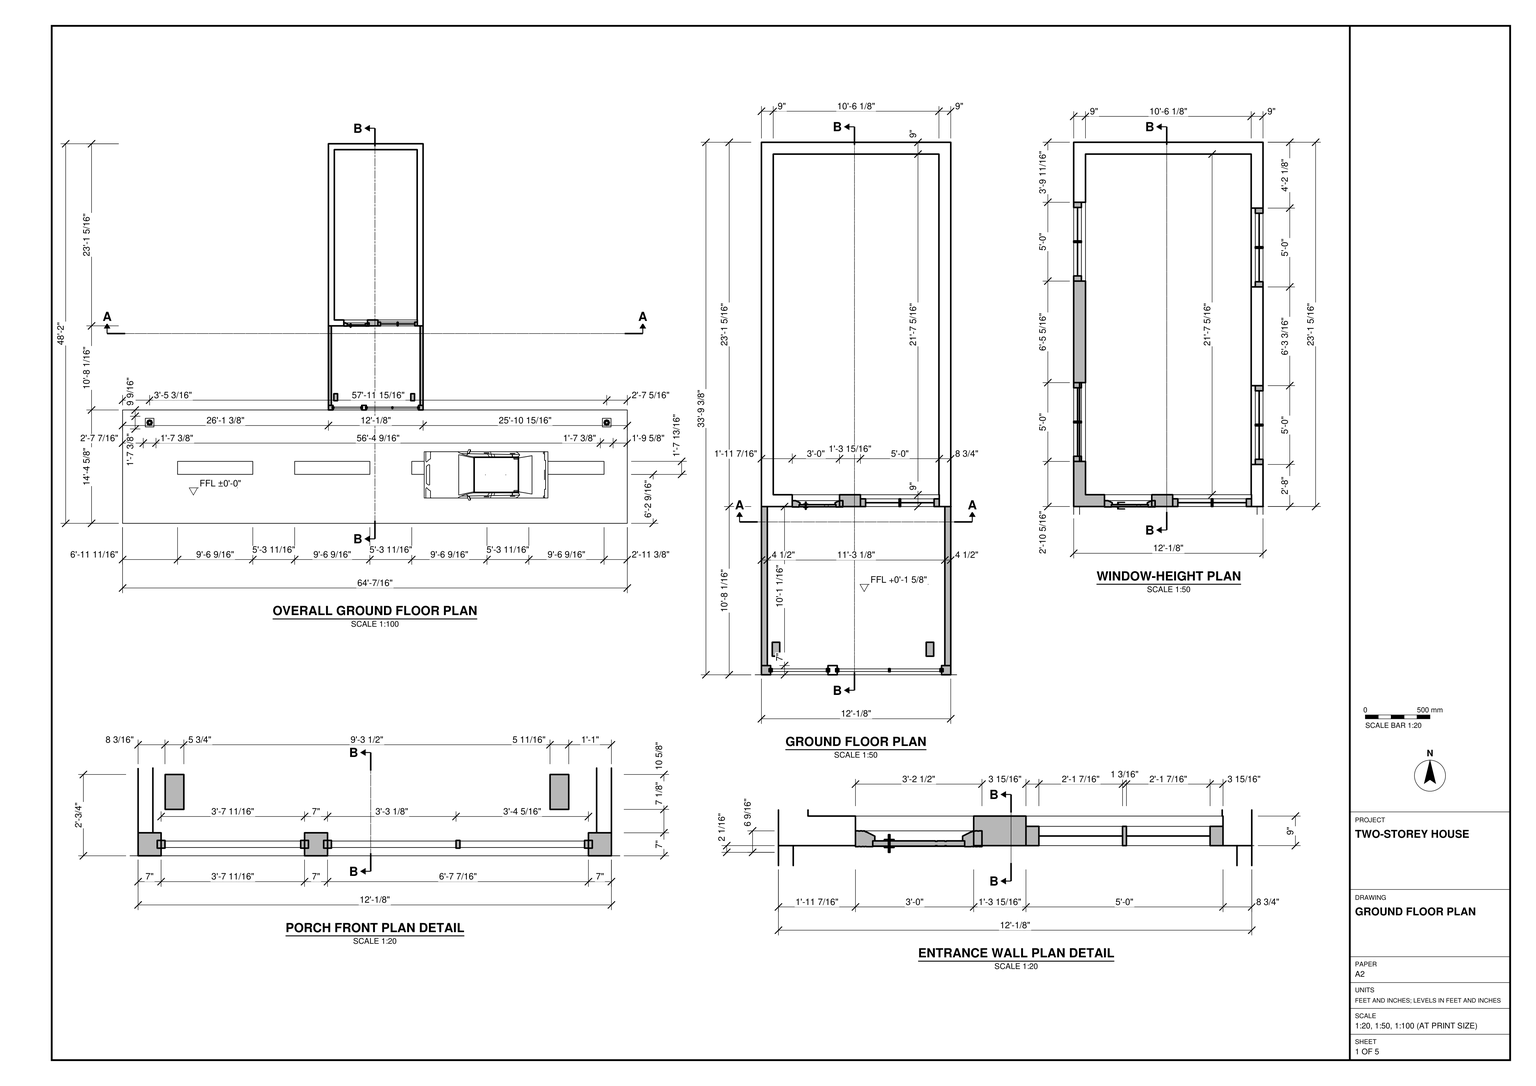
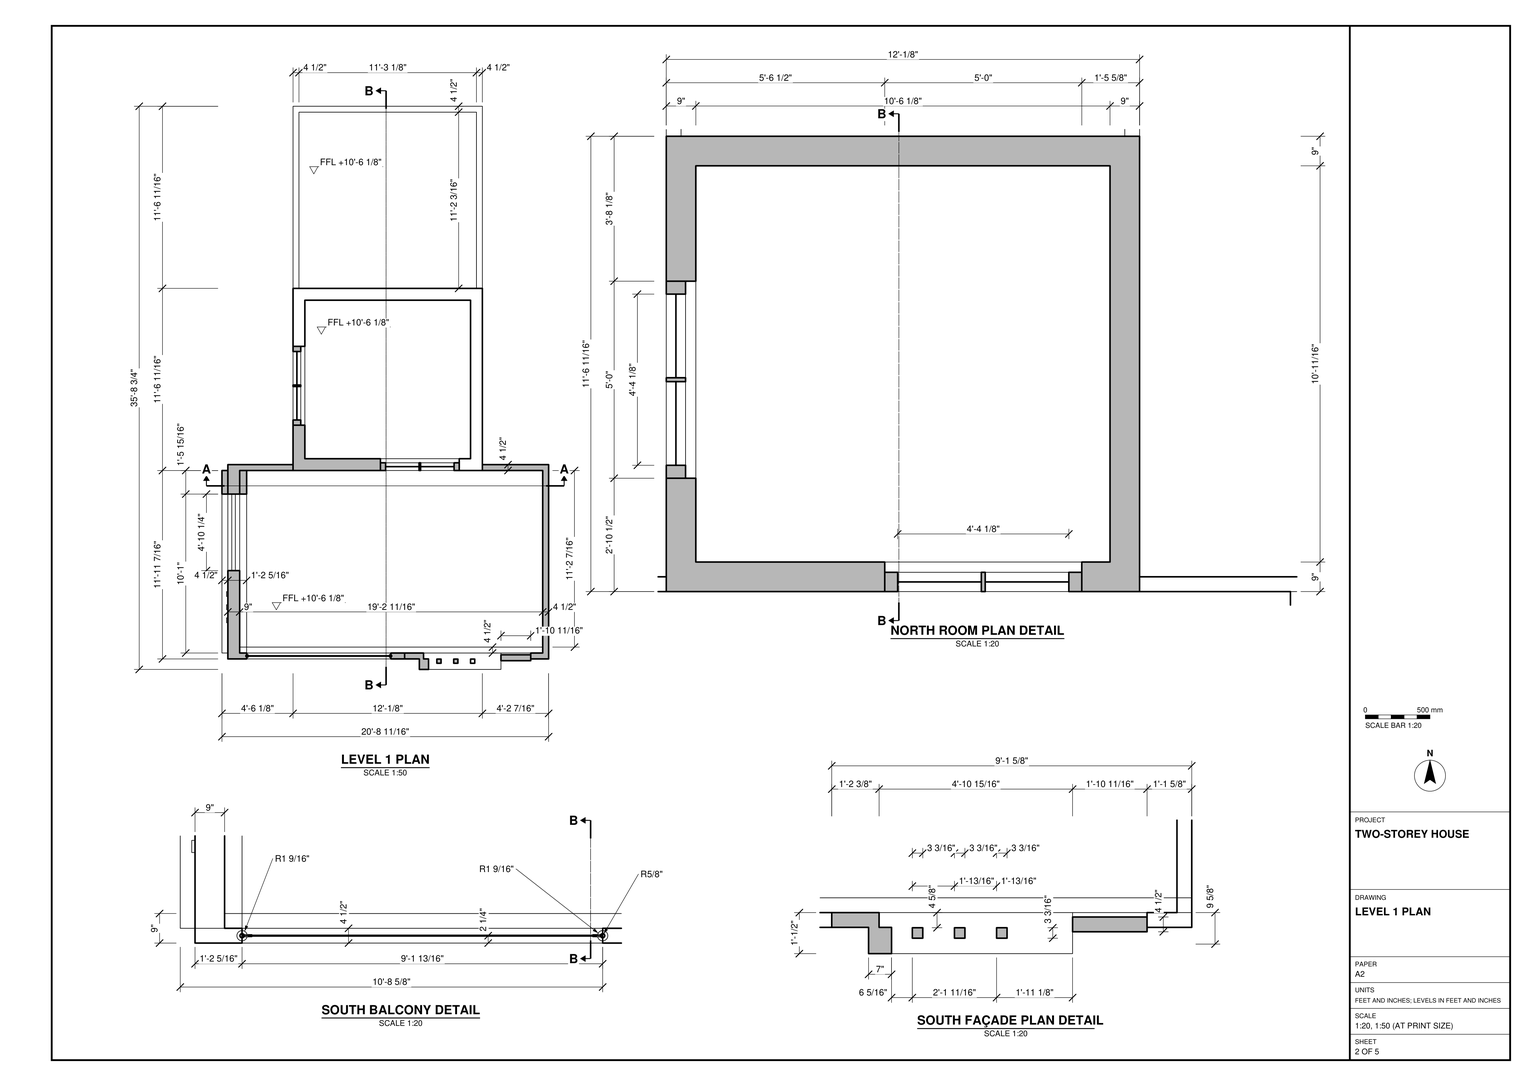
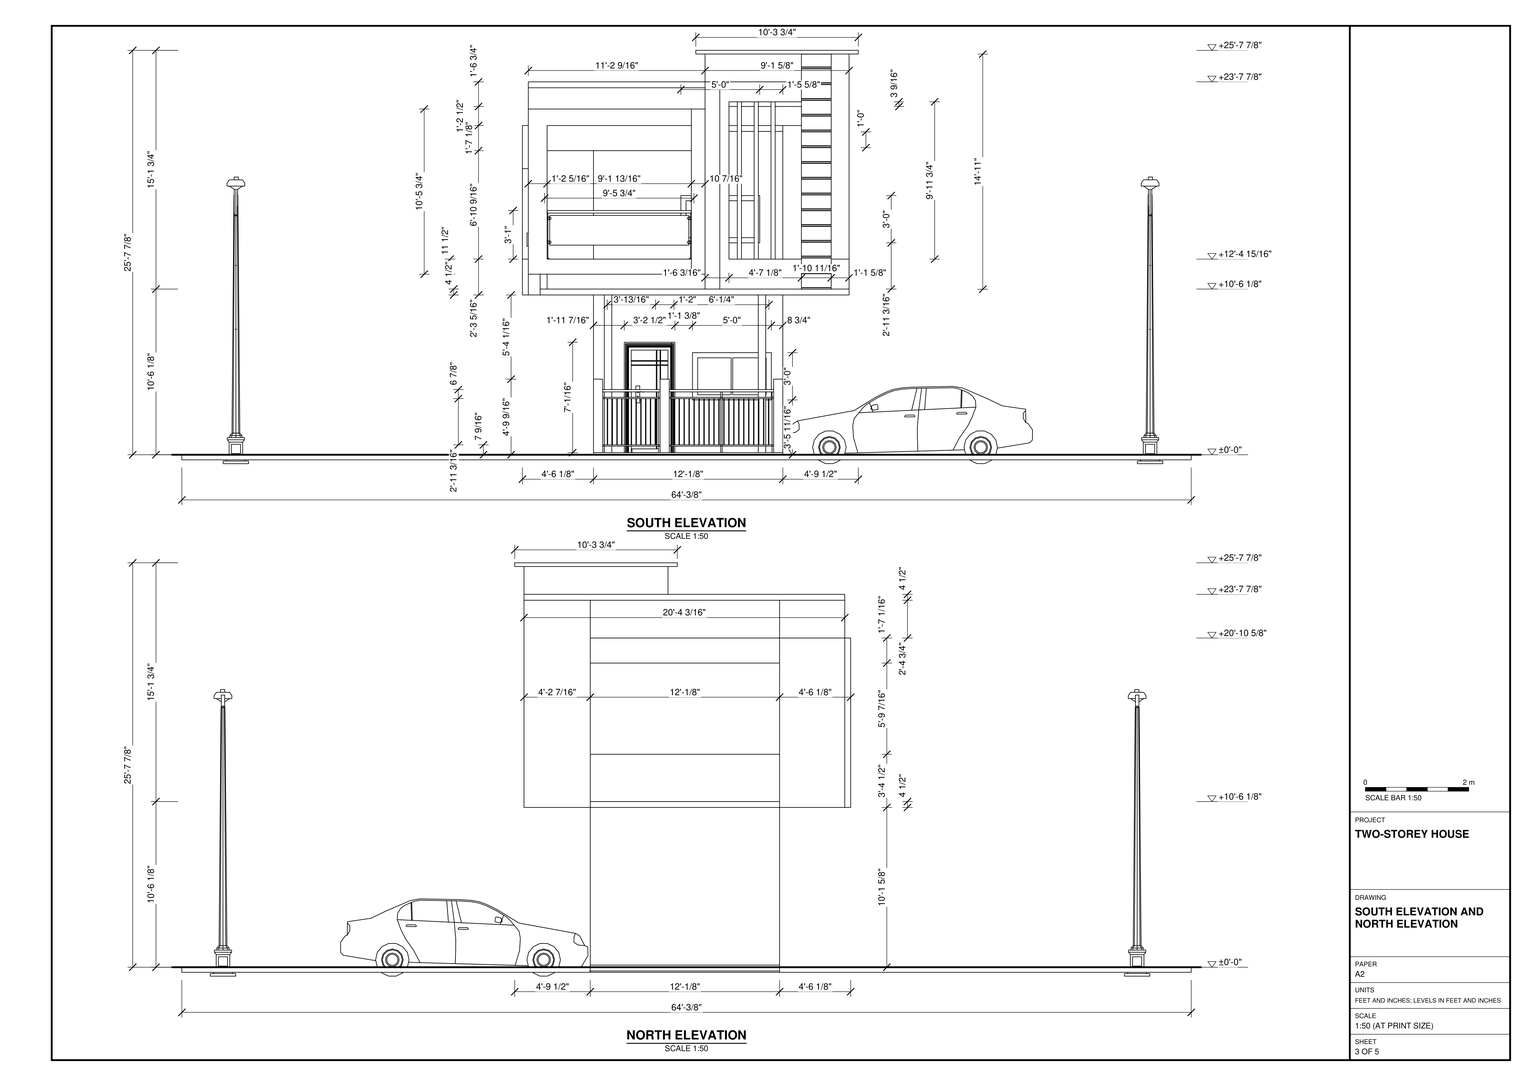
Build the house and its street frontage in SketchUp from task_files/diagram_01.pdf. Work in feet and inches. The complete model, including the street, shall measure 64'-7/16" along X, 48'-2" along Y and 26'-2 11/16" along Z. Use ±0'-0" as the ground-floor datum and +10'-6 1/8" as the upper-floor level.

Set the narrow ground-floor room perpendicular to the street, with the covered porch between the entrance wall and the road. Model the slabs, the 9" room walls, the framed door and windows, and the porch posts and railing. Use the window-height plan to locate the openings along both sides. On the upper floor, extend the wider south portion beyond both sides of the porch and retain the narrower room and terrace to the north. Follow the plan details for wall and parapet thicknesses. Reproduce the recessed south balcony, its guard, the adjacent vertical façade members and horizontal bands, and the stepped flat roofline.

Include the road markings, the car and the street lamps in the positions shown. Decor and loose items may be any suitable library components. Keep shell elements such as walls, slabs and roofs, and each furniture or joinery piece shown, in separate groups or components; use components for repeated parts. Save one SketchUp model as output_files/two_storey_house_with_a_balcony_and_street_frontage.skp.

# SketchUp Ruby script. Lengths in inches.
U = 1.inch
M = Sketchup.active_model
def pt(a) = Geom::Point3d.new(a.map { |v| v * U })
def face(e, loops, mat)
  f = e.add_face(loops[0].map { |a| pt(a) })
  loops[1..].each { |l| e.add_face(l.map { |a| pt(a) }).erase! }
  f.material = f.back_material = mat if mat
  f
end
# faces: each face lists its corners as indices into pts; further lists are holes
def faces(e, pts, list, mat = nil) = list.each { |f| face(e, (f[0].is_a?(Array) ? f : [f]).map { |l| l.map { |i| pts[i] } }, mat) }
# xy, xz, yz: faces in a plane at the given z, y or x. An outline is a flat list of corners, or four numbers for a rectangle; further outlines are holes
def ring(l) = l.size == 4 ? [[l[0], l[1]], [l[2], l[1]], [l[2], l[3]], [l[0], l[3]]] : l.each_slice(2).to_a
def flat(e, list, mat, &to3) = list.each { |f| face(e, (f[0].is_a?(Array) ? f : [f]).map { |l| ring(l).map { |u, v| to3.(u, v) } }, mat) }
def xy(e, z, list, mat = nil) = flat(e, list, mat) { |x, y| [x, y, z] }
def xz(e, y, list, mat = nil) = flat(e, list, mat) { |x, z| [x, y, z] }
def yz(e, x, list, mat = nil) = flat(e, list, mat) { |y, z| [x, y, z] }
def lines(e, pts, list) = list.each { |a, b| e.add_line(pt(pts[a]), pt(pts[b])) }
# prism: a flat outline (further loops are holes) pulled along v
def prism(e, loops, v, mat = nil)
  f = face(e, loops, mat); d = Geom::Vector3d.new(v.map { |x| x * U })
  f.pushpull(f.normal.samedirection?(d) ? d.length : -d.length)
end
def box(e, o, s, mat = nil) = prism(e, [[o, [o[0] + s[0], o[1], o[2]], [o[0] + s[0], o[1] + s[1], o[2]], [o[0], o[1] + s[1], o[2]]]], [0, 0, s[2]], mat)
def at(x, y, z, deg = 0) = Geom::Transformation.translation(pt([x, y, z])) * Geom::Transformation.rotation(ORIGIN, Z_AXIS, deg.degrees)
def axes(o, x, y, z) = Geom::Transformation.new([*x, 0, *y, 0, *z, 0, *pt(o).to_a, 1])
def part(name) = M.definitions.add(name)
# library, detail: a bought-in or finely detailed component or shape, given as its bounding box
def library(name, o, s) = part(name).tap { |d| box(d.entities, o, s) }
def detail(e, o, s) = box(e.add_group.entities, o, s)
def put(e, d, t, mat = nil) = e.add_instance(d, t).tap { |i| i.material = mat if mat }
def group(e, t, mat = nil) = e.add_group.tap { |g| g.transformation = t; g.material = mat if mat }.entities
root = M.entities
M.materials.add(" ").color = [155, 105, 61]
M.materials.add("[Blacktop Old 01]").color = [132, 136, 139]
M.materials.add("[Color B02]").color = [255, 178, 153]
M.materials.add("[Color C07]").color = [153, 76, 0]
M.materials.add("[Color G03]").color = [101, 255, 101]
M.materials.add("[Color L04]").color = [255, 50, 152]
M.materials.add("[Color M09]").color = [0, 0, 0]
M.materials.add("[Formica Beige]").color = [211, 187, 149]
M.materials.add("[Formica Blue]").color = [71, 97, 152]
M.materials.add("[Roofing Shingles Multi]").color = [136, 127, 125]
M.materials.add("[Terrazzo Light Blue]").color = [196, 214, 227]
M.materials.add("[Translucent Glass Blue]").color = [100, 149, 237]
M.materials["[Translucent Glass Blue]"].alpha = 0.5
M.materials.add("[Wood Bamboo]").color = [177, 105, 43]
M.materials.add("[Wood Floor Dark]").color = [153, 94, 42]
M.materials.add("[Wood OSB]").color = [240, 195, 122]
M.materials.add("white1").color = [255, 255, 255]
c1 = part("LampFlag")
xy(c1.entities,-0.375,[[-0.5,0,0.5,24]])
xy(c1.entities,48.25,[[-0.5,0,0.5,24]])
yz(c1.entities,0,[[3.04,0,20.96,48]])
c2 = part("LampPost")
xy(c2.entities,184.57,[[4.68,3.18,5.74,3.62,6.18,4.68,5.74,5.74,4.68,6.18,3.62,5.74,3.18,4.68,3.62,3.62]])
xy(c2.entities,185.69,[[4.68,3.64,5.41,3.95,5.72,4.68,5.41,5.41,4.68,5.72,3.95,5.41,3.64,4.68,3.72,4.5,3.95,3.95]])
p = [[4.68,0,1.5625],[1.37,1.37,1.5625],[1.37,1.37,0],[4.68,0,0],[7.99,1.37,1.5625],[7.99,1.37,0],
  [0,4.68,1.5625],[0,4.68,0],[9.36,4.68,1.5625],[9.36,4.68,0],[1.37,7.99,1.5625],[1.37,7.99,0],
  [7.99,7.99,1.5625],[7.99,7.99,0],[4.68,9.36,1.5625],[4.68,9.36,0],[4.68,1.68,3.4375],[2.56,2.56,3.4375],
  [6.8,2.56,3.4375],[1.68,4.68,3.4375],[7.68,4.68,3.4375],[2.56,6.8,3.4375],[6.8,6.8,3.4375],[4.68,7.68,3.4375],
  [4.68,3.18,184.57],[3.62,3.62,184.57],[5.74,3.62,184.57],[3.18,4.68,184.57],[6.18,4.68,184.57],[3.62,5.74,184.57],
  [5.74,5.74,184.57],[4.68,6.18,184.57],[4.68,3.64,185.69],[3.95,3.95,185.69],[5.41,3.95,185.69],[3.72,4.5,185.69],
  [3.64,4.68,185.69],[5.72,4.68,185.69],[3.95,5.41,185.69],[5.41,5.41,185.69],[4.68,5.72,185.69]]
faces(c2.entities,p,[[0,1,2,3],[4,0,3,5],[1,6,7,2],[8,4,5,9],[6,10,11,7],[12,8,9,13],[10,14,15,11],[14,12,13,15],
  [0,16,17,1],[4,18,16,0],[1,17,19,6],[18,4,8,20],[21,10,6,19],[20,8,12,22],[23,14,10,21],[22,12,14,23],
  [16,24,25,17],[18,26,24,16],[17,25,27,19],[18,20,28,26],[27,29,21,19],[20,22,30,28],[21,29,31,23],[23,31,30,22],
  [24,32,33,25],[26,34,32,24],[33,35,36,27,25],[34,26,28,37],[27,36,38,29],[37,28,30,39],[29,38,40,31],[39,30,31,40]])
c3 = part("LampBase")
box(c3.entities,[0,0,0],[19.37,19.37,2])
xy(c3.entities,6.02,[[4.53,4.53,14.84,14.84]])
xy(c3.entities,19.85,[[3.14,3.14,16.24,16.24]])
xz(c3.entities,2.52,[[2.52,2,16.85,4.57]])
xz(c3.entities,3.14,[[3.14,18.21,16.24,19.85]])
xz(c3.entities,4.53,[[[4.53,6.02,14.84,16.43],[6.19,7.6875,13.18,14.77]],[6.19,7.6875,13.18,14.77]])
xz(c3.entities,14.84,[[[4.53,6.02,14.84,16.43],[6.19,7.6875,13.18,14.77]],[6.19,7.6875,13.18,14.77]])
xz(c3.entities,16.24,[[3.14,18.21,16.24,19.85]])
xz(c3.entities,16.85,[[2.52,2,16.85,4.57]])
yz(c3.entities,2.52,[[2.52,2,16.85,4.57]])
yz(c3.entities,3.14,[[3.14,18.21,16.24,19.85]])
yz(c3.entities,4.53,[[[4.53,6.02,14.84,16.43],[6.19,7.6875,13.18,14.77]],[6.19,7.6875,13.18,14.77]])
yz(c3.entities,14.84,[[[4.53,6.02,14.84,16.43],[6.19,7.6875,13.18,14.77]],[6.19,7.6875,13.18,14.77]])
yz(c3.entities,16.24,[[3.14,18.21,16.24,19.85]])
yz(c3.entities,16.85,[[2.52,2,16.85,4.57]])
p = [[2.52,2.52,4.57],[4.53,4.53,6.02],[4.53,14.84,6.02],[2.52,16.85,4.57],[16.85,2.52,4.57],[14.84,4.53,6.02],
  [16.85,16.85,4.57],[14.84,14.84,6.02],[3.14,3.14,18.21],[3.14,16.24,18.21],[4.53,14.84,16.43],[4.53,4.53,16.43],
  [14.84,4.53,16.43],[16.24,3.14,18.21],[14.84,14.84,16.43],[16.24,16.24,18.21]]
faces(c3.entities,p,[[0,1,2,3],[4,5,1,0],[4,6,7,5],[3,2,7,6],[8,9,10,11],[12,13,8,11],[12,14,15,13],[10,9,15,14]])
c4 = part("LampFixture")
xy(c4.entities,28.375,[[9.93,5.75,6.76,6.58,6.65,6.76,6.76,6.93,9.93,7.77,13.1,6.93,13.22,6.76,13.1,6.58]],"white1")
xy(c4.entities,31,[[[9.93,0,3.28,1.74,0,6.76,3.28,11.77,9.93,13.52,16.58,11.77,25.88,8.05,25.88,5.46,16.58,1.74],[9.93,1.76,15.52,3.22,17.83,6.76,15.52,10.29,9.93,11.76,4.35,10.29,2.03,6.76,4.35,3.22]]])
xy(c4.entities,35.8,[[[9.93,1.76,15.52,3.22,17.83,6.76,15.52,10.29,9.93,11.76,4.35,10.29,2.03,6.76,4.35,3.22],[10.41,4.875,13.48,8.125]]])
xy(c4.entities,37.92,[[10.41,4.875,13.48,8.125]])
xz(c4.entities,4.875,[[10.41,35.8,13.48,37.92]])
xz(c4.entities,8.125,[[10.41,35.8,13.48,37.92]])
yz(c4.entities,10.41,[[4.875,35.8,8.125,37.92]])
yz(c4.entities,13.48,[[4.875,35.8,8.125,37.92]])
yz(c4.entities,25.88,[[5.46,31,8.05,31,8.05,33.25,7.6,33.86,6.76,33.98,5.92,33.86,5.46,33.25]])
p = [[9.93,1.76,31],[4.35,3.22,31],[6.76,6.58,28.375],[9.93,5.75,28.375],[15.52,3.22,31],[13.1,6.58,28.375],
  [2.03,6.76,31],[6.65,6.76,28.375],[17.83,6.76,31],[13.22,6.76,28.375],[4.35,10.29,31],[6.76,6.93,28.375],
  [15.52,10.29,31],[13.1,6.93,28.375],[9.93,11.76,31],[9.93,7.77,28.375],[3.28,1.74,31],[9.93,0,31],
  [9.93,0,33.25],[3.28,1.74,33.25],[16.58,1.74,31],[16.58,1.74,33.25],[0,6.76,31],[0,6.76,33.25],
  [25.88,5.46,31],[25.88,5.46,33.25],[3.28,11.77,31],[3.28,11.77,33.25],[16.58,11.77,33.25],[25.88,8.05,33.25],
  [25.88,8.05,31],[16.58,11.77,31],[9.93,13.52,31],[9.93,13.52,33.25],[9.93,1.76,35.8],[4.35,3.22,35.8],
  [15.52,3.22,35.8],[2.03,6.76,35.8],[25.88,5.92,33.86],[4.35,10.29,35.8],[15.52,10.29,35.8],[25.88,7.6,33.86],
  [9.93,11.76,35.8],[25.88,6.76,33.98],[17.83,6.76,35.8]]
faces(c4.entities,p,[[0,1,2,3],[4,0,3,5],[1,6,7,2],[8,4,5,9],[6,10,11,7],[12,8,9,13],[10,14,15,11],[14,12,13,15]],"white1")
faces(c4.entities,p,[[16,17,18,19],[17,20,21,18],[22,16,19,23],[20,24,25,21],[26,22,23,27],[28,29,30,31],[32,26,27,33],[31,32,33,28],
  [19,18,34,35],[18,21,36,34],[23,19,35,37],[21,25,38,36],[27,23,37,39],[40,41,29,28],[33,27,39,42],[28,33,42,40],
  [36,38,43,44],[44,43,41,40]])
c5 = part("StreetLamp\#1")
yz(c5.entities,99.59,[[9.6875,212.08,10.62,213.7,8.75,213.7,9.22,212.89]])
p = [[25.05,8.39,199.9],[10.46,8.39,190.22],[10.83,8.54,190.14],[11.32,9.6875,188.09],[26.14,9.6875,197.92],[10.83,10.83,190.14],
  [10.46,10.99,190.22],[25.05,10.99,199.9],[10.83,10.83,190.46],[11.3,9.6875,190.78],[10.83,8.54,190.46],[43.14,9.6875,205.5],
  [42.4,8.39,207.63],[42.4,10.99,207.63],[61.17,9.6875,210.15],[60.79,8.39,212.38],[55.1875,8.39,210.93],[48.3,9.6875,206.83],
  [55.75,9.6875,208.75],[60.79,10.99,212.38],[55.1875,10.99,210.93],[79.73,9.04,212.89],[79.68,8.39,214.01],[79.78,9.6875,211.76],
  [79.73,10.34,212.89],[79.68,10.99,214.01],[99.59,8.75,213.7],[99.59,9.6875,212.08],[99.59,9.22,212.89],[99.59,10.62,213.7],
  [42.94,9.6875,204.65],[21.15,9.6875,183.8125],[30.79,9.6875,195.63],[11.58,9.6875,154.81],[14.61,9.6875,169.92],[56.875,9.6875,210.32],
  [61.9375,9.6875,210.32]]
faces(c5.entities,p,[[0,1,2,3,4],[4,3,5,6,7],[7,6,8,9,10,1,0],[11,12,0,4],[13,11,4,7],[12,13,7,0],[14,15,16,12,11,17,18],[19,14,18,17,11,13,20],
  [15,19,20,13,12,16],[21,22,15,14,23],[24,23,14,19,25],[26,22,21,23,27,28],[27,23,24,25,29],[22,25,19,15],[26,29,25,22]])
lines(c5.entities,p,[[30,17],[31,32],[33,34],[32,30],[35,36],[34,31],[17,35]])
put(c5.entities,c1,at(35.63,9.6875,102.6875,90),"[Color M09]")
put(c5.entities,c2,at(14.37,5.01,19.85,90))
put(c5.entities,c3,at(19.37,0,0,90))
put(c5.entities,c4,at(125.47,16.44,180.3125,180))
c6 = part("Light Street 18' Decorative")
put(c6.entities,c5,at(-626.11,0,-3.625))
c7 = library("Car Sedan",[0,-0.48,0],[188.37,78.26,58.82])
c8 = part("Group1\#1")
xy(c8.entities,-4.5,[[65.875,-45.76,65.875,231.56,210,231.56,201,222.56,74.875,222.56,74.875,-36.76,89.33,-36.76,89.33,-45.76],[125.33,-45.76,125.33,-36.76,201,-36.76,201,222.56,210,231.56,210,-45.76]])
xy(c8.entities,40.09,[[141.24,-45.76,201.24,-36.76]])
xy(c8.entities,49.11,[[201.24,-13.74,210,46.26]])
xy(c8.entities,52.53,[[201.24,121.43,210,181.43]])
xy(c8.entities,56.12,[[65.875,-11.43,74.875,48.57]])
xy(c8.entities,56.4,[[65.875,125.87,74.875,185.87]])
xy(c8.entities,76.09,[[141.24,-45.76,201.24,-36.76]])
xy(c8.entities,84,[[89.33,-45.76,125.33,-36.76]])
xy(c8.entities,85.11,[[201.24,-13.74,210,46.26]])
xy(c8.entities,88.53,[[201.24,121.43,210,181.43]])
xy(c8.entities,92.12,[[65.875,-11.43,74.875,48.57]])
xy(c8.entities,92.4,[[65.875,125.87,74.875,185.87]])
xy(c8.entities,120,[[[65.875,-45.76,210,231.56],[74.875,-36.76,201,222.56]]])
xz(c8.entities,-45.76,[[[65.875,-4.5,89.33,-4.5,89.33,84,125.33,84,125.33,-4.5,210,-4.5,210,120,65.875,120],[141.24,40.09,201.24,76.09]]])
xz(c8.entities,-36.76,[[74.875,-4.5,74.875,120,201,120,201,76.09,141.24,76.09,141.24,40.09,201,40.09,201,-4.5,125.33,-4.5,125.33,84,89.33,84,89.33,-4.5]])
xz(c8.entities,-13.74,[[201.24,49.11,210,85.11]])
xz(c8.entities,-11.43,[[65.875,56.12,74.875,92.12]])
xz(c8.entities,46.26,[[201.24,49.11,210,85.11]])
xz(c8.entities,48.57,[[65.875,56.12,74.875,92.12]])
xz(c8.entities,121.43,[[201.24,52.53,210,88.53]])
xz(c8.entities,125.87,[[65.875,56.4,74.875,92.4]])
xz(c8.entities,181.43,[[201.24,52.53,210,88.53]])
xz(c8.entities,185.87,[[65.875,56.4,74.875,92.4]])
xz(c8.entities,222.56,[[74.875,-4.5,201,120]])
xz(c8.entities,231.56,[[65.875,-4.5,210,120]])
yz(c8.entities,65.875,[[[-45.76,-4.5,231.56,120],[125.87,56.4,185.87,92.4],[-11.43,56.12,48.57,92.12]]])
yz(c8.entities,74.875,[[[-36.76,-4.5,222.56,120],[125.87,56.4,185.87,92.4],[-11.43,56.12,48.57,92.12]]])
yz(c8.entities,89.33,[[-45.76,-4.5,-36.76,84]])
yz(c8.entities,125.33,[[-45.76,-4.5,-36.76,84]])
yz(c8.entities,141.24,[[-45.76,40.09,-36.76,76.09]])
yz(c8.entities,201,[[-36.76,-4.5,222.56,120]])
yz(c8.entities,201.24,[[-45.76,40.09,-36.76,76.09]])
yz(c8.entities,210,[[[-45.76,-4.5,231.56,120],[121.43,52.53,181.43,88.53],[-13.74,49.11,46.26,85.11]]])
c9 = part("Group\#12")
box(c9.entities,[0,0,0],[7,7,55.9375])
c10 = part("Group3\#1")
xy(c10.entities,124.5,[[[65.875,80.87,210,219.53],[74.875,89.87,201,210.53]]])
xy(c10.entities,159.6875,[[132.4,80.87,192.4,89.87]])
xy(c10.entities,166.54,[[65.875,115.39,74.875,175.39]])
xy(c10.entities,195.6875,[[132.4,80.87,192.4,89.87]])
xy(c10.entities,202.54,[[65.875,115.39,74.875,175.39]])
xy(c10.entities,244.5,[[[65.875,80.87,210,219.53],[74.875,89.87,201,210.53]]])
xz(c10.entities,80.87,[[[65.875,124.5,210,244.5],[132.4,159.6875,192.4,195.6875]]])
xz(c10.entities,89.87,[[[74.875,124.5,201,244.5],[132.4,159.6875,192.4,195.6875]]])
xz(c10.entities,115.39,[[65.875,166.54,74.875,202.54]])
xz(c10.entities,175.39,[[65.875,166.54,74.875,202.54]])
xz(c10.entities,210.53,[[74.875,124.5,201,244.5]])
xz(c10.entities,219.53,[[65.875,124.5,210,244.5]])
yz(c10.entities,65.875,[[[80.87,124.5,219.53,244.5],[115.39,166.54,175.39,202.54]]])
yz(c10.entities,74.875,[[[89.87,124.5,210.53,244.5],[115.39,166.54,175.39,202.54]]])
yz(c10.entities,132.4,[[80.87,159.6875,89.87,195.6875]])
yz(c10.entities,192.4,[[80.87,159.6875,89.87,195.6875]])
yz(c10.entities,201,[[89.87,124.5,210.53,244.5]])
yz(c10.entities,210,[[80.87,124.5,219.53,244.5]])
c11 = part("Group4\#2")
prism(c11.entities,[[[205.5,353.68,124.5],[70.375,353.68,124.5],[70.375,187.53,124.5],[65.875,187.53,124.5],[65.875,358.18,124.5],[210,358.18,124.5],[210,187.53,124.5],[205.5,187.53,124.5]]],[0,0,28.75])
c12 = part("Group9\#1")
box(c12.entities,[70.375,76.37,249],[135.125,4.5,28.75])
c13 = part("Group\#6")
box(c13.entities,[0,0,0],[3.1875,3.1875,119.75])
c14 = part("Group14\#1")
prism(c14.entities,[[[205.5,353.68,124.5],[70.375,353.68,124.5],[70.375,219.53,124.5],[65.875,219.53,124.5],[65.875,358.18,124.5],[210,358.18,124.5],[210,219.53,124.5],[205.5,219.53,124.5]]],[0,0,36])
c15 = part("Group\#9")
box(c15.entities,[-1,0,0],[1,3.6875,10.1875])
c16 = part("Group\#10")
box(c16.entities,[0,0,0],[2.6875,59.0625,2.1875])
c17 = part("Group18\#1")
box(c17.entities,[65.875,-40.19,0],[4.5,121.06,46.5])
c18 = part("Group\#11")
box(c18.entities,[0,0,0],[5.6875,10.625,120])
c19 = part("Group18\#2")
box(c19.entities,[65.875,-40.19,0],[4.5,121.06,46.5])
c20 = library("Group\#13",[0,0,0],[113.75,3.15,36.98])
c21 = part("Group\#16")
xy(c21.entities,0,[[0,0,79,19.8125]])
c22 = library("Group\#17",[0,-1.62,0],[36,6.12,73])
c23 = part("Group92\#1")
xy(c23.entities,0,[[-26.0625,-14.0625,-0.59,14.0625],[0.59,-14.0625,26.0625,14.0625]])
c24 = part("Group91\#1")
prism(c24.entities,[[[-30,18,0],[30,18,0],[30,-18,0],[-30,-18,0]],[[26.0625,-14.0625,0],[26.0625,14.0625,0],[0.59,14.0625,0],[0.59,-14.0625,0]],[[-26.0625,14.0625,0],[-26.0625,-14.0625,0],[-0.59,-14.0625,0],[-0.59,14.0625,0]]],[0,0,5.875]," ")
put(c24.entities,c23,at(0,0,2.9375))
c25 = part("Group93\#1")
xy(c25.entities,0,[[-26.0625,-14.0625,-0.59,14.0625],[0.59,-14.0625,26.0625,14.0625]],"[Translucent Glass Blue]")
c26 = part("Group92\#2")
prism(c26.entities,[[[30,-18,0],[-30,-18,0],[-30,18,0],[30,18,0]],[[-0.59,14.0625,0],[-26.0625,14.0625,0],[-26.0625,-14.0625,0],[-0.59,-14.0625,0]],[[26.0625,14.0625,0],[0.59,14.0625,0],[0.59,-14.0625,0],[26.0625,-14.0625,0]]],[0,0,5.875])
put(c26.entities,c25,at(0,0,2.9375))
c27 = part("Group95\#1")
xy(c27.entities,0,[[-26.0625,-14.0625,-0.59,14.0625],[0.59,-14.0625,26.0625,14.0625]],"[Translucent Glass Blue]")
c28 = part("Group94\#1")
prism(c28.entities,[[[-30,-18,0],[-30,18,0],[30,18,0],[30,-18,0]],[[-0.59,-14.0625,0],[-0.59,14.0625,0],[-26.0625,14.0625,0],[-26.0625,-14.0625,0]],[[26.0625,-14.0625,0],[26.0625,14.0625,0],[0.59,14.0625,0],[0.59,-14.0625,0]]],[0,0,5.875])
put(c28.entities,c27,at(0,0,2.9375))
c29 = part("Group97\#1")
xy(c29.entities,0,[[-26.0625,-14.0625,-0.59,14.0625],[0.59,-14.0625,26.0625,14.0625]],"[Translucent Glass Blue]")
c30 = part("Group96\#1")
prism(c30.entities,[[[-30,-18,0],[-30,18,0],[30,18,0],[30,-18,0]],[[-0.59,14.0625,0],[-26.0625,14.0625,0],[-26.0625,-14.0625,0],[-0.59,-14.0625,0]],[[0.59,-14.0625,0],[26.0625,-14.0625,0],[26.0625,14.0625,0],[0.59,14.0625,0]]],[0,0,5.875])
put(c30.entities,c29,at(0,0,2.9375))
c31 = part("Group99\#1")
xy(c31.entities,0,[[-26.0625,-14.0625,-0.59,14.0625],[0.59,-14.0625,26.0625,14.0625]],"[Translucent Glass Blue]")
c32 = part("Group98\#1")
prism(c32.entities,[[[-30,-18,0],[-30,18,0],[30,18,0],[30,-18,0]],[[-26.0625,-14.0625,0],[-0.59,-14.0625,0],[-0.59,14.0625,0],[-26.0625,14.0625,0]],[[0.59,-14.0625,0],[26.0625,-14.0625,0],[26.0625,14.0625,0],[0.59,14.0625,0]]],[0,0,5.875])
put(c32.entities,c31,at(0,0,2.9375))
c33 = part("Group101\#1")
xy(c33.entities,0,[[-26.0625,-14.0625,-0.59,14.0625],[0.59,-14.0625,26.0625,14.0625]],"[Translucent Glass Blue]")
c34 = part("Group100\#1")
prism(c34.entities,[[[30,-18,0],[-30,-18,0],[-30,18,0],[30,18,0]],[[0.59,14.0625,0],[0.59,-14.0625,0],[26.0625,-14.0625,0],[26.0625,14.0625,0]],[[-26.0625,-14.0625,0],[-0.59,-14.0625,0],[-0.59,14.0625,0],[-26.0625,14.0625,0]]],[0,0,5.875])
put(c34.entities,c33,at(0,0,2.9375))
c35 = part("Group103\#1")
xy(c35.entities,0,[[-26.0625,-14.0625,-0.59,14.0625],[0.59,-14.0625,26.0625,14.0625]],"[Translucent Glass Blue]")
c36 = part("Group102\#1")
prism(c36.entities,[[[-30,-18,0],[-30,18,0],[30,18,0],[30,-18,0]],[[-0.59,-14.0625,0],[-0.59,14.0625,0],[-26.0625,14.0625,0],[-26.0625,-14.0625,0]],[[0.59,14.0625,0],[0.59,-14.0625,0],[26.0625,-14.0625,0],[26.0625,14.0625,0]]],[0,0,5.875])
put(c36.entities,c35,at(0,0,2.9375))
c37 = part("Group125\#1")
box(c37.entities,[71.69,-44.875,0],[2.37,2.37,46.23])
c38 = part("Group126\#1")
box(c38.entities,[115.38,-44.875,0],[2.36,2.37,46.23])
c39 = part("Group128\#1")
box(c39.entities,[71.69,-45.07,46.23],[46.05,2.76,1.77])
c40 = part("Group128\#2")
box(c40.entities,[72.875,-44.68,41.11],[43.6875,1.97,0.98])
c41 = part("Group129\#1")
box(c41.entities,[72.875,-44.68,4.92],[43.6875,1.97,0.99])
c42 = part("Group130\#1")
box(c42.entities,[76.32,-44.48,5.91],[0.39,1.57,35.2])
box(c42.entities,[79.96,-44.48,5.91],[0.39,1.57,35.2])
box(c42.entities,[83.6,-44.48,5.91],[0.39,1.57,35.2])
box(c42.entities,[87.24,-44.48,5.91],[0.39,1.57,35.2])
box(c42.entities,[90.88,-44.48,5.91],[0.39,1.57,35.2])
box(c42.entities,[94.52,-44.48,5.91],[0.4,1.57,35.2])
box(c42.entities,[98.16,-44.48,5.91],[0.4,1.57,35.2])
box(c42.entities,[101.8,-44.48,5.91],[0.4,1.57,35.2])
box(c42.entities,[105.44,-44.48,5.91],[0.4,1.57,35.2])
box(c42.entities,[109.08,-44.48,5.91],[0.4,1.57,35.2])
box(c42.entities,[112.72,-44.48,5.91],[0.4,1.57,35.2])
c43 = part("Group131\#1")
box(c43.entities,[122.38,-44.875,0],[2.36,2.37,46.23])
c44 = part("Group132\#1")
box(c44.entities,[201.82,-44.875,0],[2.36,2.37,46.23])
c45 = part("Group133\#1")
box(c45.entities,[162.69,-44.875,0],[1.18,2.37,46.23])
c46 = part("Group134\#1")
box(c46.entities,[122.38,-45.07,46.23],[81.8,2.76,1.77])
c47 = part("Group135\#1")
box(c47.entities,[123.5625,-44.68,41.11],[79.4375,1.97,0.98])
c48 = part("Group136\#1")
box(c48.entities,[123.5625,-44.68,4.92],[79.4375,1.97,0.99])
c49 = part("Group137\#1")
box(c49.entities,[127.15,-44.48,5.91],[0.39,1.57,35.2])
box(c49.entities,[130.93,-44.48,5.91],[0.39,1.57,35.2])
box(c49.entities,[134.71,-44.48,5.91],[0.4,1.57,35.2])
box(c49.entities,[138.5,-44.48,5.91],[0.39,1.57,35.2])
box(c49.entities,[142.28,-44.48,5.91],[0.39,1.57,35.2])
box(c49.entities,[146.0625,-44.48,5.91],[0.4,1.57,35.2])
box(c49.entities,[149.84,-44.48,5.91],[0.4,1.57,35.2])
box(c49.entities,[153.63,-44.48,5.91],[0.39,1.57,35.2])
box(c49.entities,[157.41,-44.48,5.91],[0.39,1.57,35.2])
box(c49.entities,[161.19,-44.48,5.91],[0.4,1.57,35.2])
box(c49.entities,[164.98,-44.48,5.91],[0.39,1.57,35.2])
box(c49.entities,[168.76,-44.48,5.91],[0.39,1.57,35.2])
box(c49.entities,[172.54,-44.48,5.91],[0.39,1.57,35.2])
box(c49.entities,[176.32,-44.48,5.91],[0.4,1.57,35.2])
box(c49.entities,[180.11,-44.48,5.91],[0.39,1.57,35.2])
box(c49.entities,[183.89,-44.48,5.91],[0.39,1.57,35.2])
box(c49.entities,[187.67,-44.48,5.91],[0.4,1.57,35.2])
box(c49.entities,[191.45,-44.48,5.91],[0.4,1.57,35.2])
box(c49.entities,[195.24,-44.48,5.91],[0.39,1.57,35.2])
box(c49.entities,[199.02,-44.48,5.91],[0.39,1.57,35.2])
box(root,[313.375,466.86,229.9375],[144.125,4.5,19.0625],"[Formica Beige]")
xy(root,120,[[457.5,300.7,507.9375,305.2]])
xy(root,120,[[263.75,300.7,313.375,305.2]],"[Color B02]")
xy(root,124.5,[[480.71,161.76,507.9375,166.26],[503.4375,166.26,507.9375,300.7]])
xy(root,124.5,[[409.53,149.26,409.53,157.26,398.3125,157.26,398.3125,161.76,272.75,161.76,272.75,166.26,480.71,166.26,480.71,161.76,471.65,161.76,471.65,149.26]],"[Formica Beige]")
xy(root,135.8125,[[387.875,157.26,398.3125,161.76]],"[Color C07]")
xy(root,147.3125,[[272.75,161.76,503.4375,166.26]])
xy(root,147.3125,[[263.75,224.51,272.75,282.76]],"[Color C07]")
xy(root,147.3125,[[494.33,157.26,507.9375,161.76],[503.4375,161.76,507.9375,166.26]],"[Formica Beige]")
xy(root,147.3125,[[416.53,149.26,471.65,149.26,471.65,161.76,412.73,161.76,412.73,157.26,416.53,157.26]],"[Terrazzo Light Blue]")
xy(root,216.17,[[263.75,161.76,272.75,282.76]])
xy(root,229.875,[[278.0625,164.58,387.875,166.26]],"[Blacktop Old 01]")
xy(root,249,[[263.75,161.76,263.75,305.2,313.375,305.2,313.375,300.7,272.75,300.7,272.75,161.76],[272.75,161.76,278.0625,166.26],[278.0625,161.76,387.875,164.58],[387.875,161.76,503.4375,166.26]])
xy(root,249,[[278.0625,157.26,387.875,161.76]],"[Color C07]")
xy(root,261.5625,[[387.875,157.26,398.3125,161.76]],"[Color C07]")
xy(root,263.49,[[412.73,157.26,494.33,161.76]],"[Formica Beige]")
xy(root,267.0625,[[416.53,149.26,471.65,157.26]],"[Terrazzo Light Blue]")
xy(root,277.75,[[263.75,161.76,272.75,305.2],[272.75,166.26,272.75,300.7,313.375,300.7,313.375,305.2,457.5,305.2,457.5,300.7,503.4375,300.7,503.4375,166.26],[272.75,300.7,313.375,305.2],[457.5,300.7,503.4375,305.2]])
xy(root,282.25,[[263.75,161.76,507.9375,305.2]],"[Blacktop Old 01]")
xy(root,282.25,[[409.53,149.26,471.65,157.26]],"[Terrazzo Light Blue]")
xy(root,303.4375,[[398.3125,157.26,507.9375,161.76]])
xy(root,303.4375,[[[391.25,148.04,515,168.83],[398.3125,157.26,507.9375,161.76]]],"[Wood Floor Dark]")
xy(root,306.25,[[391.25,148.04,515,168.83]],"[Wood Floor Dark]")
xz(root,148.04,[[391.25,303.4375,515,306.25]],"[Wood Floor Dark]")
xz(root,149.26,[[409.53,124.5,471.65,124.5,471.65,147.3125,416.53,147.3125,416.53,267.0625,471.65,267.0625,471.65,282.25,409.53,282.25]],"[Terrazzo Light Blue]")
xz(root,157.26,[[412.73,127.75,416.53,147.3125],[412.73,147.3125,416.53,263.49],[409.53,267.0625,471.65,282.25]])
xz(root,157.26,[[387.875,135.8125,398.3125,261.5625]],"[Color C07]")
xz(root,157.26,[[398.3125,124.5,409.53,282.25],[494.33,147.3125,507.9375,147.3125,507.9375,303.4375,398.3125,303.4375,398.3125,282.25,471.65,282.25,471.65,267.0625,416.53,267.0625,416.53,263.49,494.33,263.49]],"[Formica Beige]")
xz(root,161.76,[[471.65,124.5,494.33,147.3125],[387.875,135.8125,398.3125,147.3125],[272.75,141.8125,278.0625,147.3125],[278.0625,141.8125,387.875,147.3125],[398.3125,147.3125,412.73,249],
  [263.75,249,272.75,253.5625],[272.75,249,387.875,253.5625],[387.875,249,398.3125,261.5625]])
xz(root,161.76,[[263.75,277.75,398.3125,282.25]],"[Blacktop Old 01]")
xz(root,161.76,[[272.75,147.3125,272.75,178.625,263.75,178.625,263.75,216.17,278.0625,216.17,278.0625,147.3125],[387.875,147.3125,398.3125,249]],"[Color C07]")
xz(root,161.76,[[272.75,124.5,398.3125,124.5,398.3125,135.8125,387.875,135.8125,387.875,141.8125,272.75,141.8125],[494.33,124.5,507.9375,147.3125],[494.33,147.3125,503.4375,249],[412.73,249,494.33,263.49],[398.3125,282.25,507.9375,303.4375]],"[Formica Beige]")
xz(root,161.76,[[263.75,253.5625,387.875,253.5625,387.875,261.5625,398.3125,261.5625,398.3125,277.75,263.75,277.75]],"[Formica Blue]")
xz(root,164.58,[[278.0625,229.875,387.875,249]],"[Blacktop Old 01]")
xz(root,166.26,[[272.75,124.5,480.71,147.3125],[480.71,124.5,503.4375,147.3125],[503.4375,124.5,507.9375,147.3125],[278.0625,229.875,278.0625,249,272.75,249,272.75,277.75,503.4375,277.75,503.4375,249,387.875,249,387.875,229.875]])
xz(root,168.83,[[391.25,303.4375,515,306.25]],"[Wood Floor Dark]")
xz(root,282.76,[[263.75,141.8125,272.75,147.3125]])
xz(root,300.7,[[272.75,249,313.375,277.75]])
xz(root,300.7,[[457.5,120,507.9375,120,507.9375,124.5,503.4375,124.5,503.4375,277.75,457.5,277.75],[272.75,124.5,313.375,249]],"[Formica Beige]")
xz(root,305.2,[[263.75,277.75,507.9375,282.25]],"[Blacktop Old 01]")
xz(root,305.2,[[263.75,120,313.375,249],[263.75,249,313.375,277.75]],"[Color B02]")
xz(root,305.2,[[457.5,120,507.9375,277.75]],"[Formica Beige]")
yz(root,263.75,[[161.76,277.75,305.2,282.25]],"[Blacktop Old 01]")
yz(root,263.75,[[300.7,120,305.2,249]],"[Color B02]")
yz(root,263.75,[[161.76,249,305.2,277.75]],"[Formica Beige]")
yz(root,272.75,[[161.76,124.5,166.26,141.8125],[161.76,141.8125,166.26,147.3125],[161.76,147.3125,166.26,178.625],[166.26,249,300.7,277.75]])
yz(root,278.0625,[[164.58,229.875,166.26,249]])
yz(root,278.0625,[[157.26,147.3125,161.76,147.3125,161.76,229.875,164.58,229.875,164.58,249,157.26,249]],"[Color C07]")
yz(root,313.375,[[300.7,120,305.2,249],[300.7,249,305.2,277.75]])
yz(root,317.875,[[335.02,56.12,395.02,92.12]])
yz(root,387.875,[[157.26,135.8125,161.76,141.8125],[157.26,141.8125,161.76,147.3125],[164.58,229.875,166.26,249],[157.26,249,161.76,253.5625],[157.26,253.5625,161.76,261.5625]])
yz(root,387.875,[[157.26,147.3125,161.76,249]],"[Color C07]")
yz(root,391.25,[[148.04,303.4375,168.83,306.25]],"[Wood Floor Dark]")
yz(root,398.3125,[[157.26,135.8125,161.76,147.3125],[157.26,147.3125,161.76,249],[157.26,249,161.76,261.5625]])
yz(root,398.3125,[[157.26,124.5,161.76,135.8125],[157.26,261.5625,161.76,282.25],[157.26,282.25,161.76,303.4375]],"[Formica Beige]")
yz(root,409.53,[[149.26,124.5,157.26,282.25]],"[Terrazzo Light Blue]")
yz(root,412.73,[[157.26,147.3125,161.76,249],[157.26,249,161.76,263.49]])
yz(root,416.53,[[149.26,147.3125,157.26,267.0625]],"[Terrazzo Light Blue]")
yz(root,457.5,[[300.7,120,305.2,277.75]])
yz(root,471.65,[[161.76,124.5,161.76,147.3125,161.11,147.3125]])
yz(root,471.65,[[149.26,124.5,161.76,124.5,161.11,147.3125,149.26,147.3125],[149.26,267.0625,157.26,282.25]],"[Terrazzo Light Blue]")
yz(root,494.33,[[157.26,147.3125,161.76,263.49]],"[Formica Beige]")
yz(root,503.4375,[[166.26,124.5,166.26,147.3125,161.76,147.3125,161.76,249,166.26,249,166.26,277.75,300.7,277.75,300.7,124.5]],"[Formica Beige]")
yz(root,507.9375,[[157.26,277.75,305.2,282.25]],"[Blacktop Old 01]")
yz(root,507.9375,[[300.7,120,305.2,120,305.2,277.75,157.26,277.75,157.26,147.3125,166.26,147.3125,166.26,124.5,300.7,124.5],[161.76,124.5,166.26,147.3125],[157.26,282.25,161.76,303.4375]],"[Formica Beige]")
yz(root,515,[[148.04,303.4375,168.83,306.25]],"[Wood Floor Dark]")
p = [[263.75,161.76,216.17],[263.75,161.76,249],[263.75,161.76,147.3125],[263.75,161.76,141.8125],[503.4375,166.26,277.75],[503.4375,161.76,277.75],
  [412.73,157.26,124.5],[412.73,157.26,127.75],[416.53,157.26,127.75],[416.53,152.76,127.75],[412.73,152.76,127.75],[494.33,157.26,282.25],
  [471.65,157.26,282.25],[458.1875,300.7,-4.5],[313.375,300.7,-4.5],[317.875,532.32,56.4],[317.875,532.32,92.4],[317.875,472.32,92.4],
  [317.875,472.32,56.4],[388.74,300.7,40.09],[388.74,300.7,76.09],[448.74,300.7,76.09],[448.74,300.7,40.09],[313.375,395.22,166.54],
  [313.375,395.22,202.54],[313.375,335.22,202.54],[313.375,335.22,166.54],[313.375,395.02,56.12],[313.375,395.02,92.12],[313.375,335.02,92.12],
  [313.375,335.02,56.12],[313.375,472.32,92.4],[313.375,532.32,92.4],[313.375,532.32,56.4],[313.375,472.32,56.4],[379.9,300.7,159.6875],
  [379.9,300.7,195.6875],[439.9,300.7,195.6875],[439.9,300.7,159.6875],[457.5,392.72,85.11],[457.5,332.72,85.11],[457.5,332.72,49.11],
  [457.5,392.72,49.11],[457.5,467.89,52.53],[457.5,467.89,88.53],[457.5,527.89,88.53],[457.5,527.89,52.53]]
lines(root,p,[[0,1],[2,3],[4,5],[6,7],[8,9],[7,10],[11,12],[13,14],[15,16],[16,17],[17,18],[18,15],
  [19,20],[20,21],[21,22],[22,19],[23,24],[24,25],[25,26],[26,23],[27,28],[28,29],[29,30],[30,27],
  [31,32],[32,33],[33,34],[34,31],[35,36],[36,37],[37,38],[38,35],[39,40],[40,41],[41,42],[42,39],
  [43,44],[44,45],[45,46],[46,43]])
put(root,c6,at(31.47,-463.04,-4.82,-90))
put(root,c6,at(727.4,-463.04,-4.82,-90))
put(root,c7,at(459.23,35.21,-8.4))
put(root,c8,at(247.5,346.46,0),"[Formica Beige]")
g1 = group(root,at(313.375,300.7,0),"[Blacktop Old 01]")
xy(g1,-5.5,[[[0,-128.0625,144.125,277.3125],[9,9,135.125,268.3125]],[9,9,135.125,268.3125]])
xy(g1,0,[[[7,-128.0625,144.125,-128.0625,144.125,277.3125,0,277.3125,0,-121.0625,7,-121.0625],[9,9,135.125,268.3125]]])
xz(g1,-128.0625,[[0,-5.5,144.125,0]])
xz(g1,277.3125,[[0,-5.5,144.125,0]])
yz(g1,0,[[-128.0625,-5.5,277.3125,0]])
yz(g1,144.125,[[-128.0625,-5.5,277.3125,0]])
p = [[135.125,268.3125,0],[135.125,268.3125,-5.5],[9,268.3125,0],[9,268.3125,-5.5],[135.125,9,0],[135.125,9,-5.5],
  [9,9,0],[9,9,-5.5]]
lines(g1,p,[[0,1],[2,3],[4,5],[6,7]])
put(g1,c9,at(0,-128.0625,0),"[Color L04]")
put(g1,c9,at(137.125,-128.0625,0),"[Color L04]")
put(g1,c9,at(50.6875,-128.0625,0),"[Color L04]")
put(root,c10,at(247.5,219.83,0),"[Formica Beige]")
put(root,c11,at(247.5,113.18,124.5),"[Formica Beige]")
g2 = group(root,at(313.375,300.7,244.5),"[Blacktop Old 01]")
box(g2,[0,0,0],[144.125,166.16,4.5])
g3 = group(root,at(263.75,161.76,120),"[Blacktop Old 01]")
xy(g3,0,[[0,0,0,138.9375,49.625,138.9375,49.625,416.25,193.75,416.25,193.75,138.9375,244.1875,138.9375,244.1875,0]])
xy(g3,4.5,[[9,0,244.1875,0,244.1875,138.9375,193.75,138.9375,193.75,277.59,49.625,277.59,49.625,138.9375,9,138.9375],[49.625,277.59,193.75,416.25]])
xz(g3,0,[[9,0,244.1875,4.5]])
xz(g3,138.9375,[[9,0,49.625,4.5],[193.75,0,244.1875,4.5]])
xz(g3,416.25,[[49.625,0,193.75,4.5]])
yz(g3,49.625,[[138.9375,0,416.25,4.5]])
yz(g3,193.75,[[138.9375,0,416.25,4.5]])
yz(g3,244.1875,[[0,0,138.9375,4.5]])
put(root,c12,at(247.5,224.33,0),"[Formica Beige]")
g4 = group(root,at(263.75,157.26,141.8125),"[Color C07]")
xy(g4,-6,[[0,0,0,125.5,9,125.5,9,4.5,124.125,4.5,124.125,0]])
xy(g4,5.5,[[14.3125,0,124.125,4.5]])
xy(g4,119.75,[[0,0,124.125,4.5]])
xz(g4,0,[[0,-6,124.125,-6,124.125,5.5,14.3125,5.5,14.3125,107.1875,124.125,107.1875,124.125,119.75,0,119.75]])
xz(g4,4.5,[[9,-6,124.125,0],[0,111.75,9,119.75],[9,111.75,124.125,119.75]])
xz(g4,125.5,[[0,-6,9,0]])
yz(g4,0,[[0,-6,4.5,119.75],[4.5,-6,125.5,0]])
yz(g4,9,[[4.5,-6,9,0],[9,-6,125.5,0]])
yz(g4,124.125,[[0,-6,4.5,5.5],[0,111.75,4.5,119.75]])
p = [[0,4.5,0],[0,0,0],[124.125,4.5,0],[124.125,0,0]]
lines(g4,p,[[0,1],[2,3]])
put(root,c13,at(422.85,153.96,147.3125),"[Wood Bamboo]")
g5 = group(root,at(263.75,161.76,120),"[Terrazzo Light Blue]")
xy(g5,0,[[-4.5,0,0,138.9375]])
xy(g5,4.5,[[9,0,14.3125,138.9375]])
xy(g5,27.3125,[[-4.5,0,0,121],[9,0,14.3125,121]])
xy(g5,96.17,[[-4.5,0,0,121],[9,0,14.3125,121]])
xy(g5,129,[[-4.5,0,0,138.9375],[9,0,14.3125,138.9375]])
xz(g5,0,[[-4.5,0,9,0,9,4.5,14.3125,4.5,14.3125,27.3125,-4.5,27.3125],[-4.5,96.17,14.3125,129]])
xz(g5,121,[[-4.5,27.3125,14.3125,96.17]])
xz(g5,138.9375,[[-4.5,0,0,129],[9,4.5,14.3125,129]])
yz(g5,-4.5,[[0,0,0,27.3125,121,27.3125,121,96.17,0,96.17,0,129,138.9375,129,138.9375,0]])
yz(g5,0,[[0,0,138.9375,0,138.9375,129,0,129,0,96.17,121,96.17,121,27.3125,0,27.3125]])
yz(g5,9,[[0,4.5,0,27.3125,121,27.3125,121,96.17,0,96.17,0,129,138.9375,129,138.9375,4.5]])
yz(g5,14.3125,[[0,4.5,138.9375,4.5,138.9375,129,0,129,0,96.17,121,96.17,121,27.3125,0,27.3125]])
put(root,c13,at(435.68,153.96,147.3125),"[Wood Bamboo]")
put(root,c13,at(448.51,153.96,147.3125),"[Wood Bamboo]")
g6 = group(root,at(471.65,157.26,124.5),"[Color C07]")
yz(g6,0,[[0.5,-0.11,0.47,1.12,-0.02,0.87,-0.34,11.87,0.17,11.62,0.125,13.12,-0.37,12.87,-0.65,22.68,3.85,22.8125,4.5,0],[-0.65,22.68,-0.68,23.87,-0.17,23.62,-0.22,25.12,-0.71,24.87,-1.02,35.87,-0.52,35.62,-0.56,37.12,-1.05,36.87,-1.36,47.87,-0.86,47.62,-0.9,49.12,-1.39,48.87,-1.71,59.87,-1.2,59.62,-1.24,61.12,-1.74,60.87,-2.05,71.87,-1.54,71.62,-1.59,73.12,-2.08,72.87,-2.39,83.87,-1.88,83.62,-1.93,85.12,-2.42,84.87,-2.73,95.87,-2.23,95.62,-2.27,97.12,-2.76,96.87,-3.08,107.87,-2.57,107.62,-2.61,109.12,-3.1,108.87,-3.42,119.87,-2.91,119.62,-2.95,121.12,-3.45,120.87,-3.76,131.87,-3.25,131.62,-3.3,133.12,-3.79,132.87,-4.1,143.87,-3.6,143.62,-3.64,145.12,-4.13,144.87,-4.45,155.87,-3.9375,155.62,-3.98,157.12,-4.47,156.87,-4.79,167.87,-4.28,167.62,-4.32,169.12,-4.82,168.87,-5.1,178.86,-0.61,178.99,3.85,22.8125]])
yz(g6,22.68,[[0.5,-0.11,4.5,0,-0.61,178.99,-5.1,178.86,-4.82,168.87,-4.32,169.12,-4.28,167.62,-4.79,167.87,-4.47,156.87,-3.98,157.12,-3.9375,155.62,-4.45,155.87,-4.13,144.87,-3.64,145.12,-3.6,143.62,-4.1,143.87,-3.79,132.87,-3.3,133.12,-3.25,131.62,-3.76,131.87,-3.45,120.87,-2.95,121.12,-2.91,119.62,-3.42,119.87,-3.1,108.87,-2.61,109.12,-2.57,107.62,-3.08,107.87,-2.76,96.87,-2.27,97.12,-2.23,95.62,-2.73,95.87,-2.42,84.87,-1.93,85.12,-1.88,83.62,-2.39,83.87,-2.08,72.87,-1.59,73.12,-1.54,71.62,-2.05,71.87,-1.74,60.87,-1.24,61.12,-1.2,59.62,-1.71,59.87,-1.39,48.87,-0.9,49.12,-0.86,47.62,-1.36,47.87,-1.05,36.87,-0.56,37.12,-0.52,35.62,-1.02,35.87,-0.71,24.87,-0.22,25.12,-0.17,23.62,-0.68,23.87,-0.37,12.87,0.125,13.12,0.17,11.62,-0.34,11.87,-0.02,0.87,0.47,1.12]])
p = [[0,0.5,-0.11],[0,4.5,0],[22.68,4.5,0],[22.68,0.5,-0.11],[22.68,0,-0.13],[0,0,-0.13],
  [22.68,0.47,1.12],[0,0.47,1.12],[0,0.5,-0.13],[22.68,0.5,-0.13],[0,3.85,22.8125],[0,-0.61,178.99],
  [22.68,-0.61,178.99],[0,-0.02,0.87],[22.68,-0.02,0.87],[22.68,-0.34,11.87],[0,-0.34,11.87],[22.68,0.17,11.62],
  [0,0.17,11.62],[22.68,0.125,13.12],[0,0.125,13.12],[0,-0.37,12.87],[22.68,-0.37,12.87],[22.68,-0.68,23.87],
  [0,-0.68,23.87],[0,-0.65,22.68],[22.68,-0.17,23.62],[0,-0.17,23.62],[22.68,-0.22,25.12],[0,-0.22,25.12],
  [22.68,-1.02,35.87],[0,-1.02,35.87],[0,-0.71,24.87],[22.68,-0.71,24.87],[22.68,-0.52,35.62],[0,-0.52,35.62],
  [22.68,-0.56,37.12],[0,-0.56,37.12],[22.68,-1.36,47.87],[0,-1.36,47.87],[0,-1.05,36.87],[22.68,-1.05,36.87],
  [22.68,-0.86,47.62],[0,-0.86,47.62],[22.68,-0.9,49.12],[0,-0.9,49.12],[22.68,-1.71,59.87],[0,-1.71,59.87],
  [0,-1.39,48.87],[22.68,-1.39,48.87],[22.68,-1.2,59.62],[0,-1.2,59.62],[22.68,-1.24,61.12],[0,-1.24,61.12],
  [22.68,-2.05,71.87],[0,-2.05,71.87],[0,-1.74,60.87],[22.68,-1.74,60.87],[22.68,-1.54,71.62],[0,-1.54,71.62],
  [22.68,-1.59,73.12],[0,-1.59,73.12],[22.68,-2.39,83.87],[0,-2.39,83.87],[0,-2.08,72.87],[22.68,-2.08,72.87],
  [22.68,-1.88,83.62],[0,-1.88,83.62],[22.68,-1.93,85.12],[0,-1.93,85.12],[22.68,-2.73,95.87],[0,-2.73,95.87],
  [0,-2.42,84.87],[22.68,-2.42,84.87],[22.68,-2.23,95.62],[0,-2.23,95.62],[22.68,-2.27,97.12],[0,-2.27,97.12],
  [22.68,-3.08,107.87],[0,-3.08,107.87],[0,-2.76,96.87],[22.68,-2.76,96.87],[22.68,-2.57,107.62],[0,-2.57,107.62],
  [22.68,-2.61,109.12],[0,-2.61,109.12],[22.68,-3.42,119.87],[0,-3.42,119.87],[0,-3.1,108.87],[22.68,-3.1,108.87],
  [22.68,-2.91,119.62],[0,-2.91,119.62],[22.68,-2.95,121.12],[0,-2.95,121.12],[22.68,-3.76,131.87],[0,-3.76,131.87],
  [0,-3.45,120.87],[22.68,-3.45,120.87],[22.68,-3.25,131.62],[0,-3.25,131.62],[22.68,-3.3,133.12],[0,-3.3,133.12],
  [22.68,-4.1,143.87],[0,-4.1,143.87],[0,-3.79,132.87],[22.68,-3.79,132.87],[22.68,-3.6,143.62],[0,-3.6,143.62],
  [22.68,-3.64,145.12],[0,-3.64,145.12],[22.68,-4.45,155.87],[0,-4.45,155.87],[0,-4.13,144.87],[22.68,-4.13,144.87],
  [22.68,-3.9375,155.62],[0,-3.9375,155.62],[22.68,-3.98,157.12],[0,-3.98,157.12],[22.68,-4.79,167.87],[0,-4.79,167.87],
  [0,-4.47,156.87],[22.68,-4.47,156.87],[22.68,-4.28,167.62],[0,-4.28,167.62],[22.68,-4.32,169.12],[0,-4.32,169.12],
  [0,-4.82,168.87],[22.68,-4.82,168.87],[22.68,-5.1,178.86],[0,-5.1,178.86]]
faces(g6,p,[[0,1,2,3,4,5],[6,7,0,8,9,3],[1,10,11,12,2],[13,14,15,16],[7,6,14,13],[16,15,17,18],[18,17,19,20],[21,22,23,24,25],
  [20,19,22,21],[26,27,24,23],[28,29,27,26],[30,31,32,33],[33,32,29,28],[34,35,31,30],[36,37,35,34],[38,39,40,41],
  [41,40,37,36],[42,43,39,38],[44,45,43,42],[46,47,48,49],[49,48,45,44],[50,51,47,46],[52,53,51,50],[54,55,56,57],
  [57,56,53,52],[58,59,55,54],[60,61,59,58],[62,63,64,65],[65,64,61,60],[66,67,63,62],[68,69,67,66],[70,71,72,73],
  [73,72,69,68],[74,75,71,70],[76,77,75,74],[78,79,80,81],[81,80,77,76],[82,83,79,78],[84,85,83,82],[86,87,88,89],
  [89,88,85,84],[90,91,87,86],[92,93,91,90],[94,95,96,97],[97,96,93,92],[98,99,95,94],[100,101,99,98],[102,103,104,105],
  [105,104,101,100],[106,107,103,102],[108,109,107,106],[110,111,112,113],[113,112,109,108],[114,115,111,110],[116,117,115,114],[118,119,120,121],
  [121,120,117,116],[122,123,119,118],[124,125,123,122],[126,127,128,129],[127,126,125,124],[12,11,129,128]])
put(root,c14,at(247.5,219.83,0),"[Formica Beige]")
g7 = group(root,at(263.75,161.76,141.8125),"[Wood OSB]")
xy(g7,36.8125,[[0,0,9,62.75]])
xz(g7,62.75,[[0,5.5,9,36.8125]])
yz(g7,0,[[0,5.5,62.75,36.8125]])
yz(g7,9,[[4.5,0,121,0,121,5.5,62.75,5.5,62.75,36.8125,4.5,36.8125]])
put(root,c15,at(263.75,204.81,156.98),"[Color G03]")
put(root,c15,at(263.75,194.83,156.98),"[Color G03]")
put(root,c15,at(263.75,184.84,156.98),"[Color G03]")
put(root,c16,at(266.75,224.51,168.51),"[Color M09]")
put(root,c16,at(266.75,224.51,161.51),"[Color M09]")
put(root,c16,at(266.75,224.51,154.51),"[Color M09]")
put(root,c17,at(247.5,219.83,0),"[Formica Beige]")
put(root,c18,at(321.62,186.77,0),"[Roofing Shingles Multi]")
put(root,c18,at(438.82,186.77,0),"[Roofing Shingles Multi]")
put(root,c19,at(387.125,219.83,0),"[Formica Beige]")
put(root,c20,at(276.09,157.9375,147.3125))
g8 = group(root,at(0,0,-5.5))
xy(g8,0,[[[0,0,768.41,172.64],[13.05,9,755.36,163.64]]])
xy(g8,3.875,[[0,0,768.41,172.64]],"[Color M09]")
xz(g8,0,[[0,0,768.41,3.875]],"[Color M09]")
xz(g8,172.64,[[0,0,768.41,3.875]],"[Color M09]")
yz(g8,0,[[0,0,172.64,3.875]],"[Color M09]")
yz(g8,768.41,[[0,0,172.64,3.875]],"[Color M09]")
p = [[13.05,9,0],[13.05,9,3.875],[755.36,163.64,0],[755.36,163.64,3.875],[755.36,9,0],[755.36,9,3.875]]
lines(g8,p,[[0,1],[2,3],[4,5]])
g9 = group(g8,at(83.7,74.57,3.875))
xy(g9,0,[[0,0,114.55,19.8125]])
put(g8,c21,axes([261.96,74.57,3.875],[1.45,0,0],[0,1,0],[0,0,1]))
put(g8,c21,axes([440.22,74.57,3.875],[1.45,0,0],[0,1,0],[0,0,1]))
put(g8,c21,axes([618.48,74.57,3.875],[1.45,0,0],[0,1,0],[0,0,1]))
put(root,c22,axes([336.83,300.39,-4.92],[1.07,0,0],[0,1.07,0],[0,0,1.2181]))
put(root,c24,axes([418.74,306.58,58.09],[1,0,0],[0,0,1],[0,-1,0]))
put(root,c26,axes([319.25,502.32,74.4],[0,-1,0],[0,0,1],[-1,0,0])," ")
put(root,c28,axes([319.25,365.22,184.54],[0,-1,0],[0,0,1],[-1,0,0])," ")
put(root,c30,axes([319.25,365.02,74.12],[0,-1,0],[0,0,1],[-1,0,0])," ")
put(root,c32,axes([409.9,306.58,177.6875],[1,0,0],[0,0,1],[0,-1,0])," ")
put(root,c34,axes([451.625,362.72,67.11],[0,1,0],[0,0,1],[1,0,0])," ")
put(root,c36,axes([451.625,497.89,70.53],[0,1,0],[0,0,1],[1,0,0])," ")
put(root,c37,at(247.5,219.83,0),"[Color M09]")
put(root,c38,at(247.5,219.83,0),"[Color M09]")
put(root,c39,at(247.5,219.83,0),"[Color M09]")
put(root,c40,at(247.5,219.83,0),"[Color M09]")
put(root,c41,at(247.5,219.83,0),"[Color M09]")
put(root,c42,at(247.5,219.83,0),"[Color C07]")
put(root,c43,at(247.5,219.83,0),"[Color M09]")
put(root,c44,at(247.5,219.83,0),"[Color M09]")
put(root,c45,at(247.5,219.83,0),"[Color M09]")
put(root,c46,at(247.5,219.83,0),"[Color M09]")
put(root,c47,at(247.5,219.83,0),"[Color M09]")
put(root,c48,at(247.5,219.83,0),"[Color M09]")
put(root,c49,at(247.5,219.83,0),"[Color C07]")
